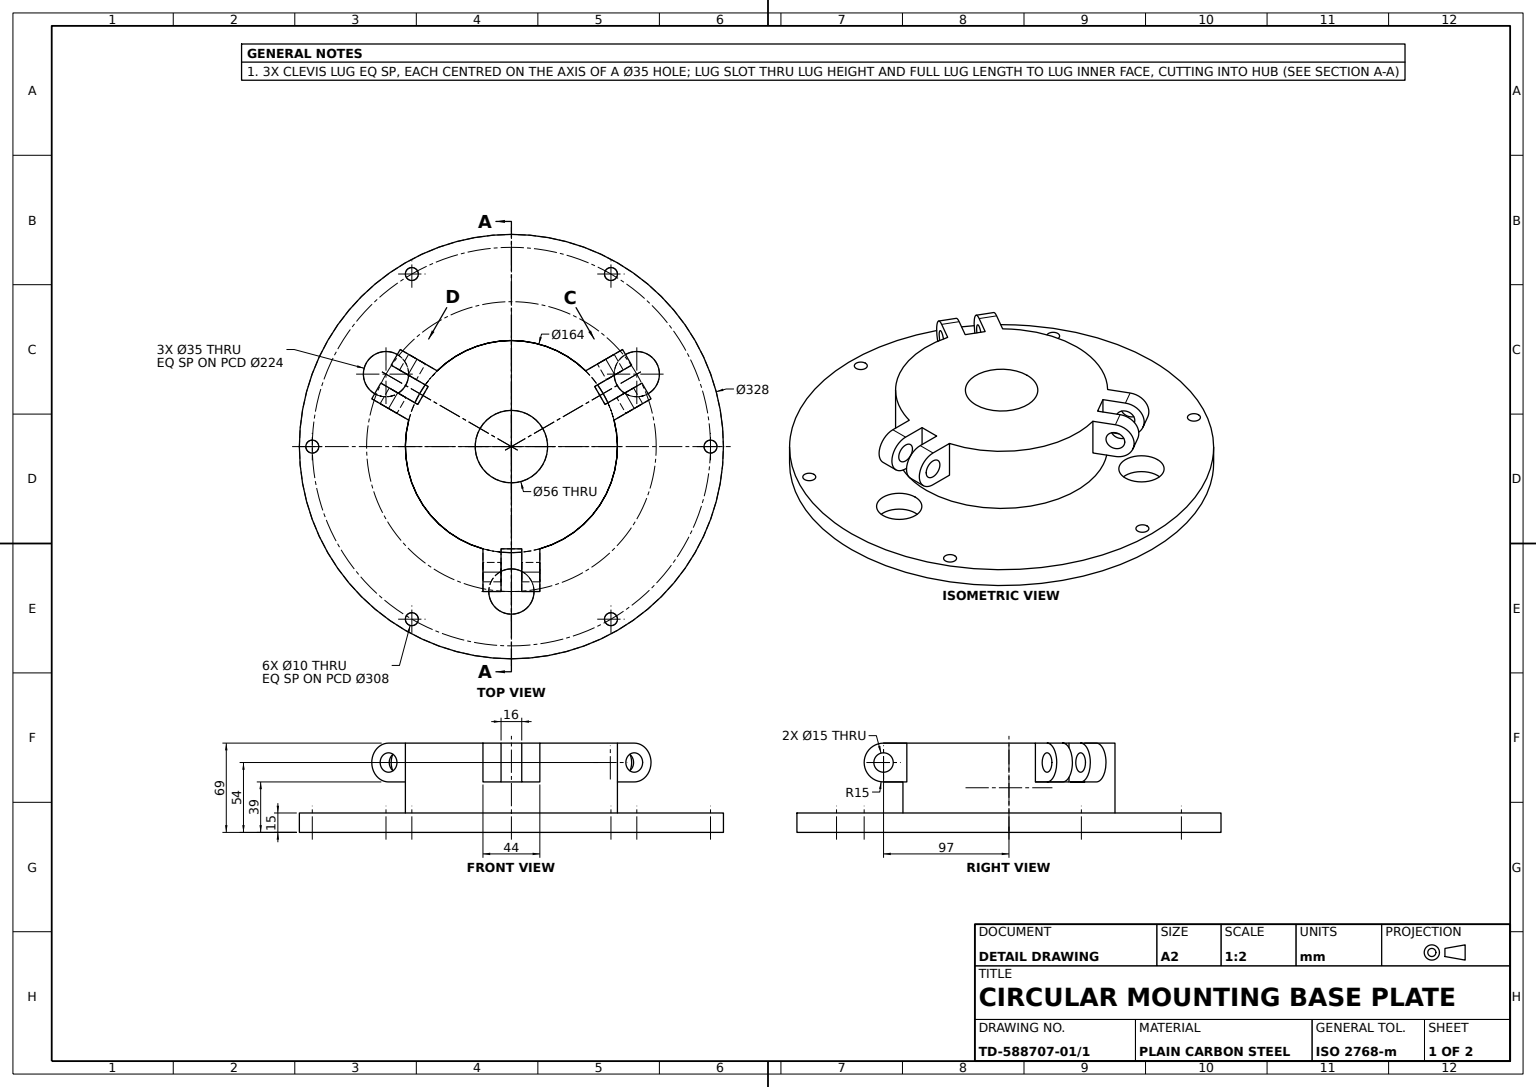
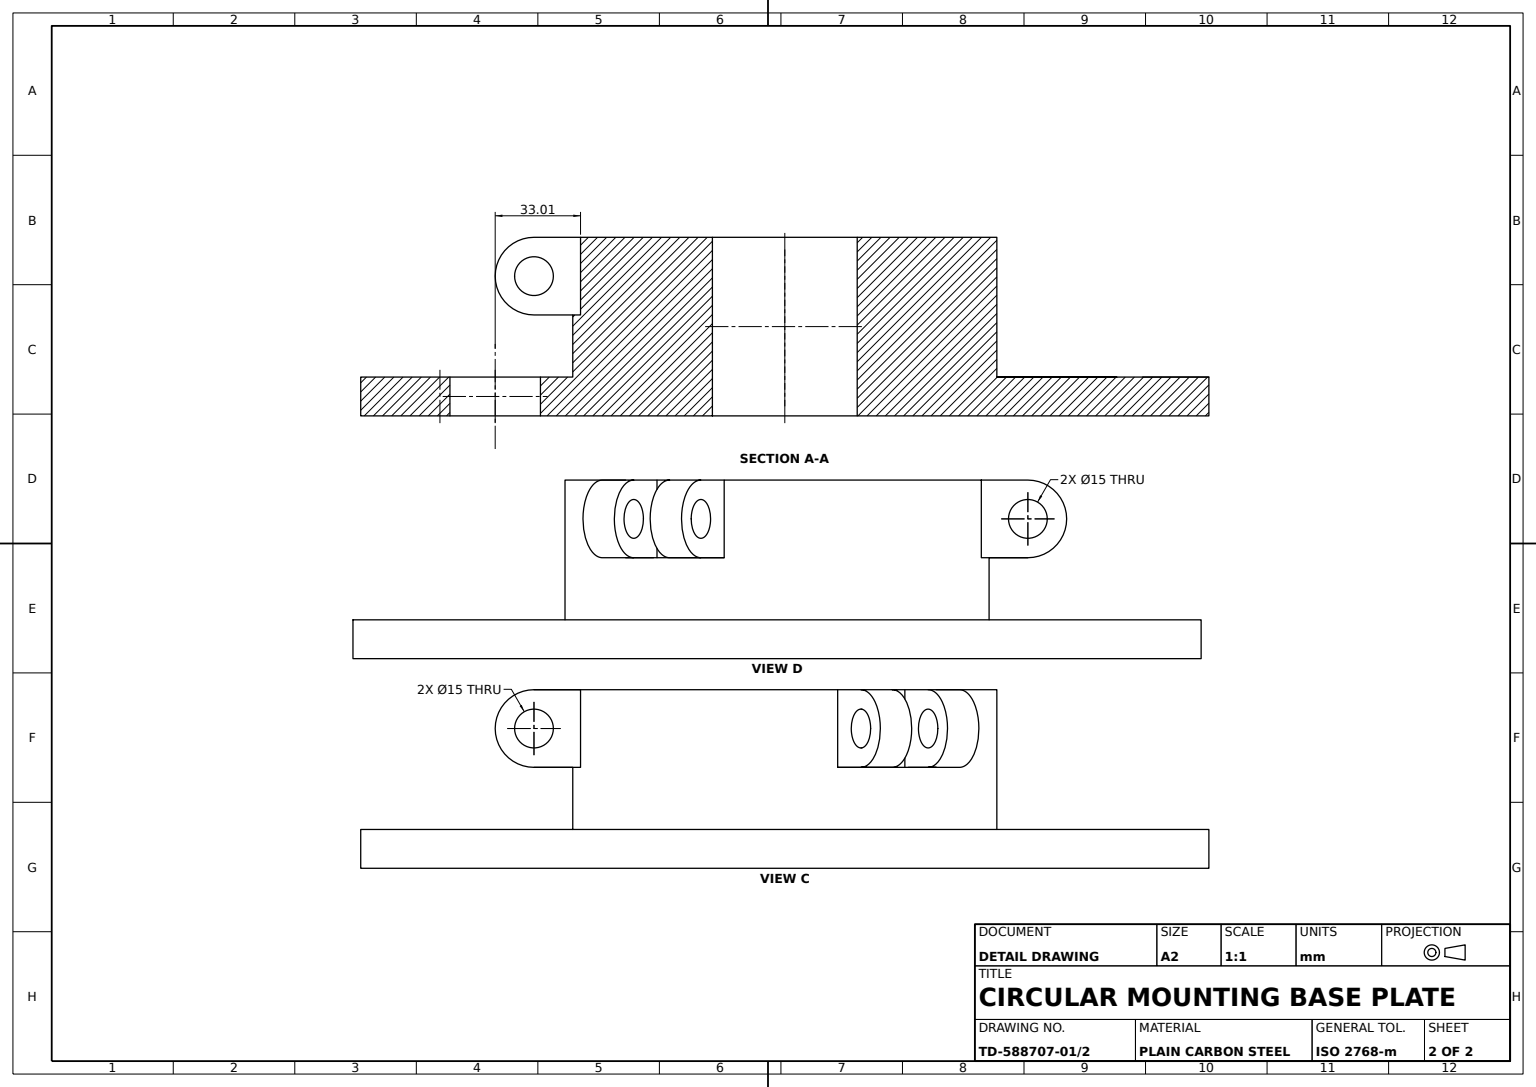
solid
v1 (72.410526,39,-32.568632)
v2 (74.675314,39,-33.876208)
e1 v1 v2 LINE
v3 (66.675314,39,-47.732615)
e2 v2 v3 CIRCLE(AX(P(0,39,0),D(0,1,0),D(0,0,1)),82)
v4 (64.410526,39,-46.425039)
e3 v3 v4 LINE
e4 v4 v1 LINE
face PLANE(AX(P(0,39,0),D(0,-1,0),D(-0.866025404,0,0.5))) rev [e1 e2 e3 e4]
v5 (-96.994845,15,-38.5)
v6 (-96.994845,15,-73.5)
e5 v5 v6 CIRCLE(AX(P(-96.994845,15,-56),D(0,1,0),D(-0.866025404,0,-0.5)),17.5)
v7 (-96.994845,0,-73.5)
e6 v7 v6 LINE
v8 (-96.994845,0,-38.5)
e7 v8 v7 CIRCLE(AX(P(-96.994845,0,-56),D(0,1,0),D(-0.866025404,0,-0.5)),17.5)
e8 v8 v5 LINE
face CYL(AX(P(-96.994845,0,-56),D(0,1,0),D(0,0,1)),17.5) rev [e5 -e6 -e7 e8]
v9 (-154,0,5)
v10 (-154,0,-5)
e9 v9 v10 CIRCLE(AX(P(-154,0,0),D(0,1,0),D(0,0,1)),5)
v11 (-154,15,5)
e10 v9 v11 LINE
v12 (-154,15,-5)
e11 v11 v12 CIRCLE(AX(P(-154,15,0),D(0,1,0),D(0,0,1)),5)
e12 v10 v12 LINE
face CYL(AX(P(-154,0,0),D(0,1,0),D(0,0,1)),5) rev [-e9 e10 e11 -e12]
v13 (77,15,138.367912)
v14 (77,15,128.367912)
e13 v13 v14 CIRCLE(AX(P(77,15,133.367912),D(0,1,0),D(0,0,1)),5)
v15 (77,0,128.367912)
e14 v15 v14 LINE
v16 (77,0,138.367912)
e15 v16 v15 CIRCLE(AX(P(77,0,133.367912),D(0,1,0),D(0.866025404,0,-0.5)),5)
e16 v16 v13 LINE
face CYL(AX(P(77,0,133.367912),D(0,1,0),D(0,0,1)),5) rev [e13 -e14 -e15 e16]
v17 (-88.004464,69,-41.571797)
v18 (-72.410526,69,-32.568632)
e17 v17 v18 LINE
v19 (-72.410526,39,-32.568632)
e18 v19 v18 LINE
v20 (-74.675314,39,-33.876208)
e19 v20 v19 LINE
v21 (-88.004464,39,-41.571797)
e20 v21 v20 LINE
v22 (-100.994845,54,-49.071797)
e21 v22 v21 CIRCLE(AX(P(-88.004464,54,-41.571797),D(-0.5,0,0.866025404),D(0.866025404,0,0.5)),15)
e22 v17 v22 CIRCLE(AX(P(-88.004464,54,-41.571797),D(-0.5,0,0.866025404),D(0.866025404,0,0.5)),15)
v23 (-81.509274,54,-37.821797)
v24 (-94.499655,54,-45.321797)
e23 v23 v24 CIRCLE(AX(P(-88.004464,54,-41.571797),D(-0.5,0,0.866025404),D(0.866025404,0,0.5)),7.5)
e24 v24 v23 CIRCLE(AX(P(-88.004464,54,-41.571797),D(-0.5,0,0.866025404),D(0.866025404,0,0.5)),7.5)
face PLANE(AX(P(-72.410526,39,-32.568632),D(-0.5,0,0.866025404),D(0.866025404,0,0.5))) rev [e17 -e18 -e19 -e20 -e21 -e22] [e23 e24]
v25 (154,15,5)
v26 (154,15,-5)
e25 v25 v26 CIRCLE(AX(P(154,15,0),D(0,1,0),D(0,0,1)),5)
v27 (154,0,-5)
e26 v27 v26 LINE
v28 (154,0,5)
e27 v28 v27 CIRCLE(AX(P(154,0,0),D(0,1,0),D(0,0,-1)),5)
e28 v28 v25 LINE
face CYL(AX(P(154,0,0),D(0,1,0),D(0,0,1)),5) rev [e25 -e26 -e27 e28]
v29 (80.004464,39,-55.428203)
e29 v29 v3 LINE
v30 (57.410526,39,-58.549394)
e30 v3 v30 CIRCLE(AX(P(0,39,0),D(0,1,0),D(0,0,1)),82)
v31 (73.004464,39,-67.552559)
e31 v31 v30 LINE
e32 v31 v29 LINE
face PLANE(AX(P(49.109297,39,-53.756678),D(0,1,0),D(0,0,1))) rev [e29 e30 -e31 e32]
v32 (72.410526,69,-32.568632)
e33 v1 v32 LINE
v33 (64.410526,69,-46.425039)
e34 v4 v33 LINE
e35 v33 v32 LINE
face PLANE(AX(P(72.410526,39,-32.568632),D(-0.866025404,0,0.5),D(0.5,0,0.866025404))) rev [-e33 -e4 e34 e35]
v34 (79.410526,39,-20.444276)
e36 v34 v2 CIRCLE(AX(P(0,39,0),D(0,1,0),D(0,0,1)),82)
v35 (88.004464,39,-41.571797)
e37 v2 v35 LINE
v36 (95.004464,39,-29.447441)
e38 v35 v36 LINE
e39 v36 v34 LINE
face PLANE(AX(P(49.109297,39,-53.756678),D(0,1,0),D(0,0,1))) rev [e36 e37 e38 e39]
v37 (-107.994845,54,-36.947441)
e40 v37 v22 LINE
v38 (-95.004464,39,-29.447441)
e41 v38 v21 LINE
e42 v37 v38 CIRCLE(AX(P(-95.004464,54,-29.447441),D(-0.5,0,0.866025404),D(0.866025404,0,0.5)),15)
face CYL(AX(P(-95.004464,54,-29.447441),D(0.5,0,-0.866025404),D(-0.866025404,0,-0.5)),15) [e40 e21 -e41 -e42]
v39 (8,69,97)
v40 (8,69,78.993671)
e43 v39 v40 LINE
v41 (8,39,78.993671)
e44 v41 v40 LINE
v42 (8,39,81.608823)
e45 v42 v41 LINE
v43 (8,39,97)
e46 v43 v42 LINE
v44 (8,54,112)
e47 v44 v43 CIRCLE(AX(P(8,54,97),D(1,0,0),D(0,0,-1)),15)
e48 v39 v44 CIRCLE(AX(P(8,54,97),D(1,0,0),D(0,0,-1)),15)
v45 (8,54,89.5)
v46 (8,54,104.5)
e49 v45 v46 CIRCLE(AX(P(8,54,97),D(1,0,0),D(0,0,-1)),7.5)
e50 v46 v45 CIRCLE(AX(P(8,54,97),D(1,0,0),D(0,0,-1)),7.5)
face PLANE(AX(P(8,39,78.993671),D(1,0,0),D(0,0,-1))) rev [e43 -e44 -e45 -e46 -e47 -e48] [e49 e50]
v47 (-95.004464,69,-29.447441)
e51 v47 v17 LINE
e52 v47 v37 CIRCLE(AX(P(-95.004464,54,-29.447441),D(-0.5,0,0.866025404),D(0.866025404,0,0.5)),15)
face CYL(AX(P(-95.004464,54,-29.447441),D(0.5,0,-0.866025404),D(-0.866025404,0,-0.5)),15) [e51 e22 -e40 -e52]
v48 (-8,69,78.993671)
e53 v40 v48 LINE
v49 (-8,39,78.993671)
e54 v49 v48 LINE
e55 v41 v49 LINE
face PLANE(AX(P(-8,39,78.993671),D(0,0,-1),D(-1,0,0))) rev [e53 -e54 -e55 e44]
v50 (22,69,97)
e56 v50 v39 LINE
v51 (22,54,112)
e57 v51 v44 LINE
e58 v50 v51 CIRCLE(AX(P(22,54,97),D(1,0,0),D(0,0,-1)),15)
face CYL(AX(P(22,54,97),D(-1,0,0),D(0,0,1)),15) [e56 e48 -e57 -e58]
e59 v12 v11 CIRCLE(AX(P(-154,15,0),D(0,1,0),D(0,0,1)),5)
e60 v10 v9 CIRCLE(AX(P(-154,0,0),D(0,1,0),D(0,0,1)),5)
face CYL(AX(P(-154,0,0),D(0,1,0),D(0,0,1)),5) rev [e12 e59 -e10 -e60]
v52 (-80.004464,39,-55.428203)
v53 (-92.994845,54,-62.928203)
e61 v52 v53 CIRCLE(AX(P(-80.004464,54,-55.428203),D(0.5,0,-0.866025404),D(-0.866025404,0,-0.5)),15)
v54 (-85.994845,54,-75.052559)
e62 v53 v54 LINE
v55 (-73.004464,39,-67.552559)
e63 v54 v55 CIRCLE(AX(P(-73.004464,54,-67.552559),D(-0.5,0,0.866025404),D(0.866025404,0,0.5)),15)
e64 v52 v55 LINE
face CYL(AX(P(-95.004464,54,-29.447441),D(0.5,0,-0.866025404),D(-0.866025404,0,-0.5)),15) [e61 e62 e63 -e64]
v56 (77,15,-138.367912)
v57 (77,15,-128.367912)
e65 v56 v57 CIRCLE(AX(P(77,15,-133.367912),D(0,1,0),D(0,0,1)),5)
e66 v57 v56 CIRCLE(AX(P(77,15,-133.367912),D(0,1,0),D(0,0,1)),5)
v58 (-77,15,128.367912)
v59 (-77,15,138.367912)
e67 v58 v59 CIRCLE(AX(P(-77,15,133.367912),D(0,1,0),D(0,0,1)),5)
e68 v59 v58 CIRCLE(AX(P(-77,15,133.367912),D(0,1,0),D(0,0,1)),5)
v60 (0,15,94.5)
v61 (0,15,129.5)
e69 v60 v61 CIRCLE(AX(P(0,15,112),D(0,1,0),D(0,0,1)),17.5)
e70 v61 v60 CIRCLE(AX(P(0,15,112),D(0,1,0),D(0,0,1)),17.5)
v62 (96.994845,15,-38.5)
v63 (96.994845,15,-73.5)
e71 v62 v63 CIRCLE(AX(P(96.994845,15,-56),D(0,1,0),D(0.866025404,0,-0.5)),17.5)
e72 v63 v62 CIRCLE(AX(P(96.994845,15,-56),D(0,1,0),D(0.866025404,0,-0.5)),17.5)
v64 (0,15,-82)
v65 (0,15,82)
e73 v64 v65 CIRCLE(AX(P(0,15,0),D(0,1,0),D(0,0,1)),82)
e74 v65 v64 CIRCLE(AX(P(0,15,0),D(0,1,0),D(0,0,1)),82)
e75 v6 v5 CIRCLE(AX(P(-96.994845,15,-56),D(0,1,0),D(-0.866025404,0,-0.5)),17.5)
e76 v26 v25 CIRCLE(AX(P(154,15,0),D(0,1,0),D(0,0,1)),5)
e77 v14 v13 CIRCLE(AX(P(77,15,133.367912),D(0,1,0),D(0,0,1)),5)
v66 (0,15,-164)
v67 (0,15,164)
e78 v66 v67 CIRCLE(AX(P(0,15,0),D(0,1,0),D(0,0,1)),164)
e79 v67 v66 CIRCLE(AX(P(0,15,0),D(0,1,0),D(0,0,1)),164)
v68 (-77,15,-128.367912)
v69 (-77,15,-138.367912)
e80 v68 v69 CIRCLE(AX(P(-77,15,-133.367912),D(0,1,0),D(0,0,1)),5)
e81 v69 v68 CIRCLE(AX(P(-77,15,-133.367912),D(0,1,0),D(0,0,1)),5)
face PLANE(AX(P(0,15,0),D(0,1,0),D(0,0,1))) [-e65 -e66] [-e67 -e68] [-e69 -e70] [-e71 -e72] [-e73 -e74] [-e5 -e75] [-e76 -e25] [-e13 -e77] [e78 e79] [-e80 -e81] [-e59 -e11]
v70 (66.509274,54,-63.802559)
v71 (79.499655,54,-71.302559)
e82 v70 v71 CIRCLE(AX(P(73.004464,54,-67.552559),D(-0.5,0,-0.866025404),D(-0.866025404,0,0.5)),7.5)
e83 v71 v70 CIRCLE(AX(P(73.004464,54,-67.552559),D(-0.5,0,-0.866025404),D(-0.866025404,0,0.5)),7.5)
v72 (73.004464,69,-67.552559)
v73 (85.994845,54,-75.052559)
e84 v72 v73 CIRCLE(AX(P(73.004464,54,-67.552559),D(-0.5,0,-0.866025404),D(-0.866025404,0,0.5)),15)
e85 v73 v31 CIRCLE(AX(P(73.004464,54,-67.552559),D(-0.5,0,-0.866025404),D(-0.866025404,0,0.5)),15)
v74 (57.410526,69,-58.549394)
e86 v74 v30 LINE
e87 v74 v72 LINE
face PLANE(AX(P(73.004464,54,-67.552559),D(-0.5,0,-0.866025404),D(-0.866025404,0,0.5))) [-e82 -e83] [e84 e85 e31 -e86 e87]
v75 (22,54,89.5)
e88 v75 v45 LINE
v76 (22,54,104.5)
e89 v76 v46 LINE
e90 v76 v75 CIRCLE(AX(P(22,54,97),D(1,0,0),D(0,0,-1)),7.5)
face CYL(AX(P(22,54,97),D(-1,0,0),D(0,0,1)),7.5) rev [e88 -e50 -e89 e90]
v77 (0,39,82)
e91 v77 v42 CIRCLE(AX(P(0,39,0),D(0,1,0),D(0,0,1)),82)
v78 (-8,39,81.608823)
e92 v49 v78 LINE
e93 v78 v77 CIRCLE(AX(P(0,39,0),D(0,1,0),D(0,0,1)),82)
face PLANE(AX(P(0,39,0),D(0,-1,0),D(0,0,-1))) rev [e91 e45 e55 e92 e93]
v79 (96.994845,0,-73.5)
e94 v79 v63 LINE
v80 (96.994845,0,-38.5)
e95 v80 v62 LINE
e96 v79 v80 CIRCLE(AX(P(96.994845,0,-56),D(0,1,0),D(0.866025404,0,-0.5)),17.5)
face CYL(AX(P(96.994845,0,-56),D(0,1,0),D(0,0,1)),17.5) rev [e94 e72 -e95 -e96]
v81 (22,39,97)
e97 v51 v81 CIRCLE(AX(P(22,54,97),D(1,0,0),D(0,0,-1)),15)
v82 (22,39,78.993671)
e98 v81 v82 LINE
v83 (22,69,78.993671)
e99 v83 v82 LINE
e100 v83 v50 LINE
e101 v75 v76 CIRCLE(AX(P(22,54,97),D(1,0,0),D(0,0,-1)),7.5)
face PLANE(AX(P(22,54,97),D(1,0,0),D(0,0,-1))) [e97 e98 -e99 e100 e58] [-e90 -e101]
v84 (-8,54,104.5)
v85 (-22,54,104.5)
e102 v84 v85 LINE
v86 (-22,54,89.5)
e103 v86 v85 CIRCLE(AX(P(-22,54,97),D(1,0,0),D(0,0,-1)),7.5)
v87 (-8,54,89.5)
e104 v87 v86 LINE
e105 v84 v87 CIRCLE(AX(P(-8,54,97),D(-1,0,0),D(0,0,1)),7.5)
face CYL(AX(P(22,54,97),D(-1,0,0),D(0,0,1)),7.5) rev [e102 -e103 -e104 -e105]
v88 (92.994845,54,-62.928203)
e106 v88 v29 CIRCLE(AX(P(80.004464,54,-55.428203),D(-0.5,0,-0.866025404),D(-0.866025404,0,0.5)),15)
v89 (80.004464,69,-55.428203)
e107 v89 v88 CIRCLE(AX(P(80.004464,54,-55.428203),D(-0.5,0,-0.866025404),D(-0.866025404,0,0.5)),15)
e108 v89 v33 LINE
v90 (73.509274,54,-51.678203)
v91 (86.499655,54,-59.178203)
e109 v90 v91 CIRCLE(AX(P(80.004464,54,-55.428203),D(-0.5,0,-0.866025404),D(-0.866025404,0,0.5)),7.5)
e110 v91 v90 CIRCLE(AX(P(80.004464,54,-55.428203),D(-0.5,0,-0.866025404),D(-0.866025404,0,0.5)),7.5)
face PLANE(AX(P(64.410526,39,-46.425039),D(-0.5,0,-0.866025404),D(-0.866025404,0,0.5))) rev [-e106 -e107 e108 -e34 -e3 -e29] [e109 e110]
face CYL(AX(P(22,54,97),D(-1,0,0),D(0,0,1)),7.5) rev [-e49 -e88 e101 e89]
v92 (0,0,164)
e111 v67 v92 LINE
v93 (0,0,-164)
e112 v66 v93 LINE
e113 v93 v92 CIRCLE(AX(P(0,0,0),D(0,1,0),D(0,0,1)),164)
face CYL(AX(P(0,15,0),D(0,-1,0),D(0,0,-1)),164) [-e111 -e78 e112 e113]
v94 (-86.499655,54,-59.178203)
v95 (-79.499655,54,-71.302559)
e114 v94 v95 LINE
v96 (-66.509274,54,-63.802559)
e115 v96 v95 CIRCLE(AX(P(-73.004464,54,-67.552559),D(-0.5,0,0.866025404),D(0.866025404,0,0.5)),7.5)
v97 (-73.509274,54,-51.678203)
e116 v97 v96 LINE
e117 v94 v97 CIRCLE(AX(P(-80.004464,54,-55.428203),D(0.5,0,-0.866025404),D(-0.866025404,0,-0.5)),7.5)
face CYL(AX(P(-95.004464,54,-29.447441),D(0.5,0,-0.866025404),D(-0.866025404,0,-0.5)),7.5) rev [e114 -e115 -e116 -e117]
v98 (-77,0,-128.367912)
e118 v98 v68 LINE
v99 (-77,0,-138.367912)
e119 v99 v98 CIRCLE(AX(P(-77,0,-133.367912),D(0,1,0),D(-0.866025404,0,0.5)),5)
e120 v99 v69 LINE
face CYL(AX(P(-77,0,-133.367912),D(0,1,0),D(0,0,1)),5) rev [-e118 -e119 e120 e81]
v100 (0,69,-82)
e121 v100 v64 LINE
e122 v74 v100 CIRCLE(AX(P(0,69,0),D(0,1,0),D(0,0,1)),82)
v101 (79.410526,69,-20.444276)
e123 v101 v34 LINE
e124 v83 v101 CIRCLE(AX(P(0,69,0),D(0,1,0),D(0,0,1)),82)
e125 v42 v82 CIRCLE(AX(P(0,39,0),D(0,1,0),D(0,0,1)),82)
e126 v77 v65 LINE
face CYL(AX(P(0,69,0),D(0,-1,0),D(0,0,-1)),82) [-e121 -e122 e86 -e30 -e2 -e36 -e123 -e124 e99 -e125 -e91 e126 e74]
e127 v72 v89 LINE
e128 v73 v88 LINE
face CYL(AX(P(73.004464,54,-67.552559),D(0.5,0,0.866025404),D(0.866025404,0,-0.5)),15) [e127 e107 -e128 -e84]
e129 v92 v93 CIRCLE(AX(P(0,0,0),D(0,1,0),D(0,0,1)),164)
face CYL(AX(P(0,15,0),D(0,-1,0),D(0,0,-1)),164) [-e79 e111 e129 -e112]
v102 (88.004464,69,-41.571797)
e130 v32 v102 LINE
v103 (100.994845,54,-49.071797)
e131 v103 v102 CIRCLE(AX(P(88.004464,54,-41.571797),D(0.5,0,0.866025404),D(0.866025404,0,-0.5)),15)
e132 v35 v103 CIRCLE(AX(P(88.004464,54,-41.571797),D(0.5,0,0.866025404),D(0.866025404,0,-0.5)),15)
v104 (94.499655,54,-45.321797)
v105 (81.509274,54,-37.821797)
e133 v104 v105 CIRCLE(AX(P(88.004464,54,-41.571797),D(0.5,0,0.866025404),D(0.866025404,0,-0.5)),7.5)
e134 v105 v104 CIRCLE(AX(P(88.004464,54,-41.571797),D(0.5,0,0.866025404),D(0.866025404,0,-0.5)),7.5)
face PLANE(AX(P(100.994845,39,-49.071797),D(0.5,0,0.866025404),D(0.866025404,0,-0.5))) rev [e130 -e131 -e132 -e37 -e1 e33] [e133 e134]
v106 (-80.004464,69,-55.428203)
v107 (-73.004464,69,-67.552559)
e135 v106 v107 LINE
e136 v107 v54 CIRCLE(AX(P(-73.004464,54,-67.552559),D(-0.5,0,0.866025404),D(0.866025404,0,0.5)),15)
e137 v53 v106 CIRCLE(AX(P(-80.004464,54,-55.428203),D(0.5,0,-0.866025404),D(-0.866025404,0,-0.5)),15)
face CYL(AX(P(-95.004464,54,-29.447441),D(0.5,0,-0.866025404),D(-0.866025404,0,-0.5)),15) [e135 e136 -e62 e137]
v108 (0,0,94.5)
e138 v108 v60 LINE
v109 (0,0,129.5)
e139 v109 v61 LINE
e140 v108 v109 CIRCLE(AX(P(0,0,112),D(0,1,0),D(0,0,1)),17.5)
face CYL(AX(P(0,0,112),D(0,1,0),D(0,0,1)),17.5) rev [e138 e69 -e139 -e140]
v110 (88.509274,54,-25.697441)
v111 (101.499655,54,-33.197441)
e141 v110 v111 CIRCLE(AX(P(95.004464,54,-29.447441),D(-0.5,0,-0.866025404),D(-0.866025404,0,0.5)),7.5)
e142 v105 v110 LINE
e143 v104 v111 LINE
face CYL(AX(P(73.004464,54,-67.552559),D(0.5,0,0.866025404),D(0.866025404,0,-0.5)),7.5) rev [-e141 -e142 -e133 e143]
v112 (-8,54,112)
v113 (-22,54,112)
e144 v112 v113 LINE
v114 (-8,69,97)
e145 v112 v114 CIRCLE(AX(P(-8,54,97),D(-1,0,0),D(0,0,1)),15)
v115 (-22,69,97)
e146 v114 v115 LINE
e147 v115 v113 CIRCLE(AX(P(-22,54,97),D(1,0,0),D(0,0,-1)),15)
face CYL(AX(P(22,54,97),D(-1,0,0),D(0,0,1)),15) [-e144 e145 e146 e147]
v116 (-77,0,138.367912)
e148 v116 v59 LINE
v117 (-77,0,128.367912)
e149 v117 v116 CIRCLE(AX(P(-77,0,133.367912),D(0,1,0),D(0.866025404,0,0.5)),5)
e150 v117 v58 LINE
face CYL(AX(P(-77,0,133.367912),D(0,1,0),D(0,0,1)),5) rev [e67 -e148 -e149 e150]
e151 v97 v94 CIRCLE(AX(P(-80.004464,54,-55.428203),D(0.5,0,-0.866025404),D(-0.866025404,0,-0.5)),7.5)
e152 v95 v96 CIRCLE(AX(P(-73.004464,54,-67.552559),D(-0.5,0,0.866025404),D(0.866025404,0,0.5)),7.5)
face CYL(AX(P(-95.004464,54,-29.447441),D(0.5,0,-0.866025404),D(-0.866025404,0,-0.5)),7.5) rev [-e151 e116 -e152 -e114]
v118 (0,0,28)
v119 (0,69,28)
e153 v118 v119 LINE
v120 (0,69,-28)
e154 v119 v120 CIRCLE(AX(P(0,69,0),D(0,1,0),D(0,0,1)),28)
v121 (0,0,-28)
e155 v121 v120 LINE
e156 v118 v121 CIRCLE(AX(P(0,0,0),D(0,1,0),D(0,0,1)),28)
face CYL(AX(P(0,0,0),D(0,1,0),D(0,0,1)),28) rev [e153 e154 -e155 -e156]
v122 (-57.410526,69,-58.549394)
e157 v122 v107 LINE
v123 (-57.410526,39,-58.549394)
e158 v122 v123 LINE
e159 v55 v123 LINE
face PLANE(AX(P(-73.004464,54,-67.552559),D(-0.5,0,0.866025404),D(0.866025404,0,0.5))) rev [e152 e115] [-e63 -e136 -e157 e158 -e159]
v124 (-66.675314,39,-47.732615)
e160 v124 v52 LINE
e161 v123 v124 CIRCLE(AX(P(0,39,0),D(0,1,0),D(0,0,1)),82)
face PLANE(AX(P(-71.109297,39,-15.65156),D(0,1,0),D(0,0,1))) rev [e160 e64 e159 e161]
v125 (-22,39,78.993671)
e162 v125 v78 CIRCLE(AX(P(0,39,0),D(0,1,0),D(0,0,1)),82)
v126 (-22,69,78.993671)
e163 v126 v125 LINE
v127 (-79.410526,69,-20.444276)
e164 v127 v126 CIRCLE(AX(P(0,69,0),D(0,1,0),D(0,0,1)),82)
v128 (-79.410526,39,-20.444276)
e165 v127 v128 LINE
e166 v20 v128 CIRCLE(AX(P(0,39,0),D(0,1,0),D(0,0,1)),82)
e167 v124 v20 CIRCLE(AX(P(0,39,0),D(0,1,0),D(0,0,1)),82)
e168 v100 v122 CIRCLE(AX(P(0,69,0),D(0,1,0),D(0,0,1)),82)
face CYL(AX(P(0,69,0),D(0,-1,0),D(0,0,-1)),82) [e121 e73 -e126 -e93 -e162 -e163 -e164 e165 -e166 -e167 -e161 -e158 -e168]
v129 (77,0,-138.367912)
e169 v129 v56 LINE
v130 (77,0,-128.367912)
e170 v130 v57 LINE
e171 v129 v130 CIRCLE(AX(P(77,0,-133.367912),D(0,1,0),D(-0.866025404,0,-0.5)),5)
face CYL(AX(P(77,0,-133.367912),D(0,1,0),D(0,0,1)),5) rev [e169 e65 -e170 -e171]
e172 v15 v16 CIRCLE(AX(P(77,0,133.367912),D(0,1,0),D(0.866025404,0,-0.5)),5)
face CYL(AX(P(77,0,133.367912),D(0,1,0),D(0,0,1)),5) rev [-e16 -e172 e14 e77]
e173 v81 v43 LINE
face CYL(AX(P(22,54,97),D(-1,0,0),D(0,0,1)),15) [-e173 -e97 e57 e47]
e174 v109 v108 CIRCLE(AX(P(0,0,112),D(0,1,0),D(0,0,1)),17.5)
face CYL(AX(P(0,0,112),D(0,1,0),D(0,0,1)),17.5) rev [e139 e70 -e138 -e174]
e175 v38 v128 LINE
e176 v127 v47 LINE
v131 (-88.509274,54,-25.697441)
v132 (-101.499655,54,-33.197441)
e177 v131 v132 CIRCLE(AX(P(-95.004464,54,-29.447441),D(-0.5,0,0.866025404),D(0.866025404,0,0.5)),7.5)
e178 v132 v131 CIRCLE(AX(P(-95.004464,54,-29.447441),D(-0.5,0,0.866025404),D(0.866025404,0,0.5)),7.5)
face PLANE(AX(P(-95.004464,54,-29.447441),D(-0.5,0,0.866025404),D(0.866025404,0,0.5))) [e52 e42 e175 -e165 e176] [-e177 -e178]
e179 v87 v84 CIRCLE(AX(P(-8,54,97),D(-1,0,0),D(0,0,1)),7.5)
e180 v85 v86 CIRCLE(AX(P(-22,54,97),D(1,0,0),D(0,0,-1)),7.5)
face CYL(AX(P(22,54,97),D(-1,0,0),D(0,0,1)),7.5) rev [-e179 e104 -e180 -e102]
e181 v70 v90 LINE
e182 v71 v91 LINE
face CYL(AX(P(73.004464,54,-67.552559),D(0.5,0,0.866025404),D(0.866025404,0,-0.5)),7.5) rev [-e109 -e181 e82 e182]
e183 v98 v99 CIRCLE(AX(P(-77,0,-133.367912),D(0,1,0),D(-0.866025404,0,0.5)),5)
face CYL(AX(P(-77,0,-133.367912),D(0,1,0),D(0,0,1)),5) rev [e80 -e120 -e183 e118]
e184 v48 v114 LINE
v133 (-8,39,97)
e185 v133 v112 CIRCLE(AX(P(-8,54,97),D(-1,0,0),D(0,0,1)),15)
e186 v78 v133 LINE
face PLANE(AX(P(-8,39,112),D(-1,0,0),D(0,0,1))) rev [e179 e105] [e184 -e145 -e185 -e186 -e92 e54]
e187 v126 v115 LINE
v134 (95.004464,69,-29.447441)
e188 v101 v134 LINE
e189 v102 v134 LINE
v135 (-64.410526,69,-46.425039)
e190 v135 v106 LINE
e191 v18 v135 LINE
e192 v120 v119 CIRCLE(AX(P(0,69,0),D(0,1,0),D(0,0,1)),28)
face PLANE(AX(P(0,69,0),D(0,1,0),D(0,0,1))) [-e176 e164 e187 -e146 -e184 -e53 -e43 -e56 -e100 e124 e188 -e189 -e130 -e35 -e108 -e127 -e87 e122 e168 e157 -e135 -e190 -e191 -e17 -e51] [-e154 -e192]
v136 (-64.410526,39,-46.425039)
e193 v136 v124 LINE
e194 v136 v135 LINE
face PLANE(AX(P(-92.994845,39,-62.928203),D(0.5,0,-0.866025404),D(-0.866025404,0,-0.5))) rev [-e193 e194 e190 -e137 -e61 -e160] [e117 e151]
v137 (-22,39,97)
e195 v113 v137 CIRCLE(AX(P(-22,54,97),D(1,0,0),D(0,0,-1)),15)
e196 v133 v137 LINE
face CYL(AX(P(22,54,97),D(-1,0,0),D(0,0,1)),15) [e185 e144 e195 -e196]
e197 v19 v136 LINE
face PLANE(AX(P(0,39,0),D(0,-1,0),D(0.866025404,0,0.5))) rev [e167 e19 e197 e193]
e198 v27 v28 CIRCLE(AX(P(154,0,0),D(0,1,0),D(0,0,-1)),5)
e199 v121 v118 CIRCLE(AX(P(0,0,0),D(0,1,0),D(0,0,1)),28)
e200 v80 v79 CIRCLE(AX(P(96.994845,0,-56),D(0,1,0),D(0.866025404,0,-0.5)),17.5)
e201 v130 v129 CIRCLE(AX(P(77,0,-133.367912),D(0,1,0),D(-0.866025404,0,-0.5)),5)
e202 v116 v117 CIRCLE(AX(P(-77,0,133.367912),D(0,1,0),D(0.866025404,0,0.5)),5)
e203 v7 v8 CIRCLE(AX(P(-96.994845,0,-56),D(0,1,0),D(-0.866025404,0,-0.5)),17.5)
face PLANE(AX(P(0,0,0),D(0,1,0),D(0,0,1))) rev [e172 e15] [e198 e27] [e60 e9] [e199 e156] [e200 e96] [e174 e140] [e171 e201] [e202 e149] [e203 e7] [e119 e183] [-e129 -e113]
face CYL(AX(P(73.004464,54,-67.552559),D(0.5,0,0.866025404),D(0.866025404,0,-0.5)),15) [e128 e106 -e32 -e85]
e204 v137 v125 LINE
face PLANE(AX(P(22,39,69.408237),D(0,1,0),D(0,0,1))) rev [e162 e186 e196 e204]
face PLANE(AX(P(-22,54,97),D(1,0,0),D(0,0,-1))) rev [-e204 -e195 -e147 -e187 e163] [e180 e103]
e205 v111 v110 CIRCLE(AX(P(95.004464,54,-29.447441),D(-0.5,0,-0.866025404),D(-0.866025404,0,0.5)),7.5)
face CYL(AX(P(73.004464,54,-67.552559),D(0.5,0,0.866025404),D(0.866025404,0,-0.5)),7.5) rev [-e134 e142 -e205 -e143]
face PLANE(AX(P(-71.109297,39,-15.65156),D(0,1,0),D(0,0,1))) rev [e41 e20 e166 -e175]
v138 (107.994845,54,-36.947441)
e206 v103 v138 LINE
e207 v138 v36 CIRCLE(AX(P(95.004464,54,-29.447441),D(-0.5,0,-0.866025404),D(-0.866025404,0,0.5)),15)
face CYL(AX(P(73.004464,54,-67.552559),D(0.5,0,0.866025404),D(0.866025404,0,-0.5)),15) [-e38 e132 e206 e207]
face CYL(AX(P(96.994845,0,-56),D(0,1,0),D(0,0,1)),17.5) rev [-e200 e95 e71 -e94]
face CYL(AX(P(77,0,-133.367912),D(0,1,0),D(0,0,1)),5) rev [e170 e66 -e169 -e201]
e208 v131 v23 LINE
e209 v132 v24 LINE
face CYL(AX(P(-95.004464,54,-29.447441),D(0.5,0,-0.866025404),D(-0.866025404,0,-0.5)),7.5) rev [e178 e208 -e24 -e209]
face CYL(AX(P(73.004464,54,-67.552559),D(0.5,0,0.866025404),D(0.866025404,0,-0.5)),7.5) rev [e83 e181 -e110 -e182]
face CYL(AX(P(-77,0,133.367912),D(0,1,0),D(0,0,1)),5) rev [-e202 e148 e68 -e150]
face CYL(AX(P(154,0,0),D(0,1,0),D(0,0,1)),5) rev [e76 -e28 -e198 e26]
e210 v134 v138 CIRCLE(AX(P(95.004464,54,-29.447441),D(-0.5,0,-0.866025404),D(-0.866025404,0,0.5)),15)
face CYL(AX(P(73.004464,54,-67.552559),D(0.5,0,0.866025404),D(0.866025404,0,-0.5)),15) [e189 e210 -e206 e131]
face CYL(AX(P(0,0,0),D(0,1,0),D(0,0,1)),28) rev [e192 -e153 -e199 e155]
face CYL(AX(P(-96.994845,0,-56),D(0,1,0),D(0,0,1)),17.5) rev [e75 -e8 -e203 e6]
face PLANE(AX(P(22,39,69.408237),D(0,1,0),D(0,0,1))) rev [e125 -e98 e173 e46]
face PLANE(AX(P(95.004464,54,-29.447441),D(-0.5,0,-0.866025404),D(-0.866025404,0,0.5))) rev [-e210 -e188 e123 -e39 -e207] [e205 e141]
face CYL(AX(P(-95.004464,54,-29.447441),D(0.5,0,-0.866025404),D(-0.866025404,0,-0.5)),7.5) rev [-e208 e177 e209 -e23]
face PLANE(AX(P(-64.410526,39,-46.425039),D(0.866025404,0,0.5),D(0.5,0,-0.866025404))) rev [e18 e191 -e194 -e197]
